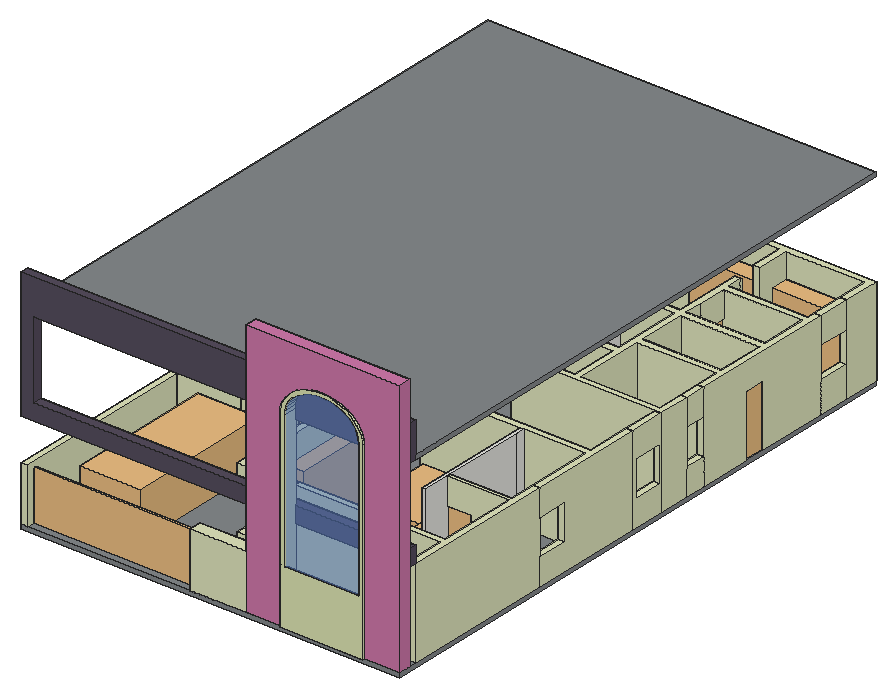
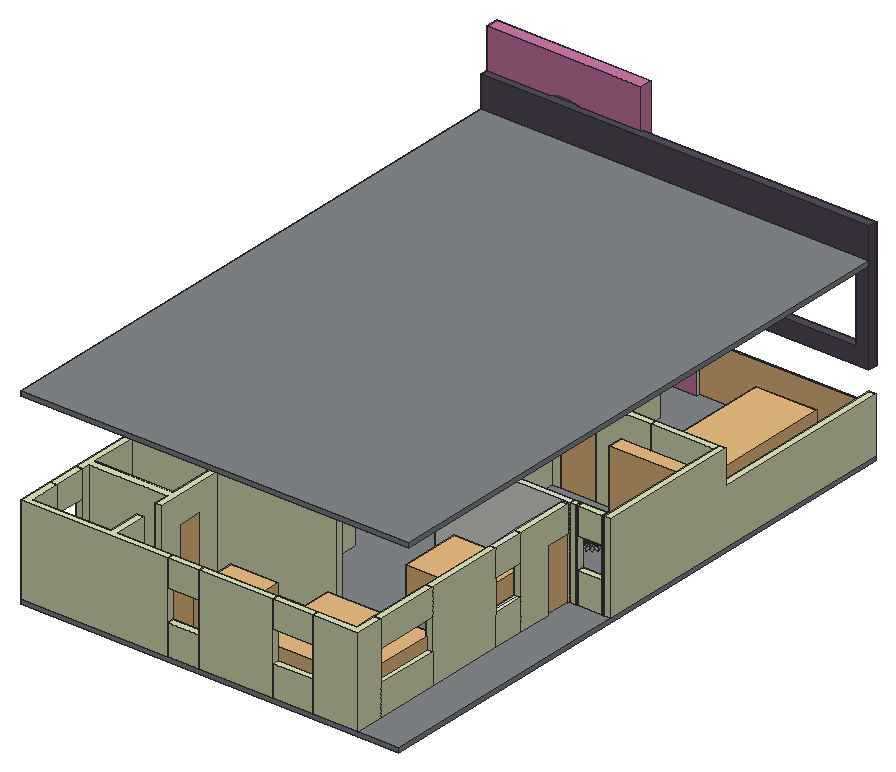
# SketchUp Ruby script. Lengths in inches.
U = 1.inch
M = Sketchup.active_model
def pt(a) = Geom::Point3d.new(a.map { |v| v * U })
def face(e, loops, mat)
  f = e.add_face(loops[0].map { |a| pt(a) })
  loops[1..].each { |l| e.add_face(l.map { |a| pt(a) }).erase! }
  f.material = f.back_material = mat if mat
  f
end
# faces: each face lists its corners as indices into pts; further lists are holes
def faces(e, pts, list, mat = nil) = list.each { |f| face(e, (f[0].is_a?(Array) ? f : [f]).map { |l| l.map { |i| pts[i] } }, mat) }
# xy, xz, yz: faces in a plane at the given z, y or x. An outline is a flat list of corners, or four numbers for a rectangle; further outlines are holes
def ring(l) = l.size == 4 ? [[l[0], l[1]], [l[2], l[1]], [l[2], l[3]], [l[0], l[3]]] : l.each_slice(2).to_a
def flat(e, list, mat, &to3) = list.each { |f| face(e, (f[0].is_a?(Array) ? f : [f]).map { |l| ring(l).map { |u, v| to3.(u, v) } }, mat) }
def xy(e, z, list, mat = nil) = flat(e, list, mat) { |x, y| [x, y, z] }
def xz(e, y, list, mat = nil) = flat(e, list, mat) { |x, z| [x, y, z] }
def yz(e, x, list, mat = nil) = flat(e, list, mat) { |y, z| [x, y, z] }
def lines(e, pts, list) = list.each { |a, b| e.add_line(pt(pts[a]), pt(pts[b])) }
# prism: a flat outline (further loops are holes) pulled along v
def prism(e, loops, v, mat = nil)
  f = face(e, loops, mat); d = Geom::Vector3d.new(v.map { |x| x * U })
  f.pushpull(f.normal.samedirection?(d) ? d.length : -d.length)
end
def box(e, o, s, mat = nil) = prism(e, [[o, [o[0] + s[0], o[1], o[2]], [o[0] + s[0], o[1] + s[1], o[2]], [o[0], o[1] + s[1], o[2]]]], [0, 0, s[2]], mat)
def at(x, y, z, deg = 0) = Geom::Transformation.translation(pt([x, y, z])) * Geom::Transformation.rotation(ORIGIN, Z_AXIS, deg.degrees)
def axes(o, x, y, z) = Geom::Transformation.new([*x, 0, *y, 0, *z, 0, *pt(o).to_a, 1])
def part(name) = M.definitions.add(name)
# library, detail: a bought-in or finely detailed component or shape, given as its bounding box
def library(name, o, s) = part(name).tap { |d| box(d.entities, o, s) }
def detail(e, o, s) = box(e.add_group.entities, o, s)
def put(e, d, t, mat = nil) = e.add_instance(d, t).tap { |i| i.material = mat if mat }
def group(e, t, mat = nil) = e.add_group.tap { |g| g.transformation = t; g.material = mat if mat }.entities
root = M.entities
M.materials.add("0206 AP 9414 PINK FLOWER").color = [207, 120, 170]
M.materials.add("0272 AP 9625 Blue Grape-N").color = [85, 77, 93]
M.materials.add("0748 AP 7713 LIME SQUASH").color = [220, 228, 179]
M.materials.add("0763 AP 7730 GREEN TOMATO").color = [223, 228, 188]
M.materials.add("0825 AP 9841 Aniseed Green-N").color = [202, 186, 112]
M.materials.add("[Blacktop Old 01]").color = [132, 136, 139]
M.materials.add("[Translucent Glass Blue]").color = [100, 149, 237]
M.materials["[Translucent Glass Blue]"].alpha = 0.5
c1 = library("michel-club1",[-34.67,-0.85,-0.13],[126.28,91.17,33.41])
c2 = library("Catia",[-24.7,0,-4.44],[60.13,63.39,38.33])
c3 = library("Mesa+de+Jantar+Clean-Ouro",[12.6875,-84.97,0.5625],[145.94,104.19,56.09])
c4 = library("toilet",[85.22,-15.77,0],[26.79,17.15,27.58])
c5 = library("bed",[0,0,0],[81.24,78.82,29.53])
c6 = library("Untitled",[0,0,0],[36,4.39,84])
c7 = part("Group\#146")
xy(c7.entities,0,[[0,0,18.2,28.93]])
xy(c7.entities,1.42,[[0.71,1.42,18.2,27.51]])
xy(c7.entities,13.47,[[0.71,1.42,18.2,27.51]])
xy(c7.entities,14.18,[[0.71,1.42,18.2,27.51]])
xy(c7.entities,25.88,[[0.71,1.42,18.2,27.51]])
xy(c7.entities,26.59,[[0.71,1.42,18.2,27.51]])
xy(c7.entities,38.65,[[0.71,1.42,18.2,27.51]])
xy(c7.entities,40.0625,[[0,0,18.2,28.93]])
xz(c7.entities,0,[[0,0,18.2,40.0625]])
xz(c7.entities,1.42,[[0.71,1.42,18.2,13.47],[0.71,14.18,18.2,25.88],[0.71,26.59,18.2,38.65]])
xz(c7.entities,27.51,[[0.71,1.42,18.2,13.47],[0.71,14.18,18.2,25.88],[0.71,26.59,18.2,38.65]])
xz(c7.entities,28.93,[[0,0,18.2,40.0625]])
yz(c7.entities,0,[[0,0,28.93,40.0625]])
yz(c7.entities,0.71,[[1.42,1.42,27.51,13.47],[1.42,14.18,27.51,25.88],[1.42,26.59,27.51,38.65]])
yz(c7.entities,18.2,[[[0,0,28.93,40.0625],[1.42,1.42,27.51,25.88],[1.42,26.59,27.51,38.65]],[1.42,13.47,27.51,14.18]])
c8 = library("tv unit model",[-7.7,0,0],[29.4,107.72,88.39])
c9 = part("*U2")
p = [[0,-10.98,0],[0.69,-9.51,0],[1.27,-7.99,0],[1.75,-6.43,0],[2.13,-4.85,0],[2.4,-3.25,0],
  [2.5625,-1.625,0],[2.62,0,0],[2.5625,1.625,0],[2.4,3.25,0],[2.13,4.85,0],[1.75,6.43,0],
  [1.27,7.99,0],[0.69,9.51,0],[0,10.98,0],[-0.69,9.51,0],[-1.27,7.99,0],[-1.75,6.43,0],
  [-2.13,4.85,0],[-2.4,3.25,0],[-2.5625,1.625,0],[-2.62,0,0],[-2.5625,-1.625,0],[-2.4,-3.25,0],
  [-2.13,-4.85,0],[-1.75,-6.43,0],[-1.27,-7.99,0],[-0.69,-9.51,0]]
lines(c9.entities,p,[[0,1],[1,2],[2,3],[3,4],[4,5],[5,6],[6,7],[7,8],[8,9],[9,10],[10,11],[11,12],
  [12,13],[13,14],[14,15],[15,16],[16,17],[17,18],[18,19],[19,20],[20,21],[21,22],[22,23],[23,24],
  [24,25],[25,26],[26,27],[27,0]])
c10 = part("*U3")
put(c10.entities,c9,at(0,11.05,0))
put(c10.entities,c9,at(-3.57,10.45,0,18.947))
put(c10.entities,c9,at(-6.74,8.73,0,37.895))
put(c10.entities,c9,at(-9.19,6.07,0,56.842))
put(c10.entities,c9,at(-10.65,2.76,0,75.789))
put(c10.entities,c9,at(-10.94,-0.84,0,94.737))
put(c10.entities,c9,at(-10.06,-4.35,0,113.684))
put(c10.entities,c9,at(-8.08,-7.37,0,132.632))
put(c10.entities,c9,at(-5.23,-9.59,0,151.579))
put(c10.entities,c9,at(-1.81,-10.77,0,170.526))
put(c10.entities,c9,at(1.81,-10.77,0,-170.526))
put(c10.entities,c9,at(5.23,-9.59,0,-151.579))
put(c10.entities,c9,at(8.08,-7.37,0,-132.632))
put(c10.entities,c9,at(10.06,-4.35,0,-113.684))
put(c10.entities,c9,at(10.94,-0.84,0,-94.737))
put(c10.entities,c9,at(10.65,2.76,0,-75.789))
put(c10.entities,c9,at(9.19,6.07,0,-56.842))
put(c10.entities,c9,at(6.74,8.73,0,-37.895))
put(c10.entities,c9,at(3.57,10.45,0,-18.947))
c11 = library("*U5",[-21.75,-13.5,0],[21,24,0.01])
c12 = library("Dining Set - 36 x 72 in.",[-45.5,-27.5,0],[91,55,0.01])
c13 = library("Range-Oven - 30 in top",[-15,-13,0],[30,26,0.01])
c14 = part("*U31")
p = [[-15.25,-21.5,0],[-17.25,-27.5,0],[-7.25,-27.5,0],[-15.25,-27.5,0]]
lines(c14.entities,p,[[0,1],[2,3]])
c15 = library("Component",[0,4.7,0],[98.27,23.62,86.61])
c16 = part("Group541\#1")
yz(c16.entities,285.5,[[630.18,36,645.93,59.625]])
c17 = library("Evoque+Azul+Marinho+As+Novinha+Fica+Loca+2017",[-10.19,-69.08,0],[168.96,82.02,63.04])
c18 = library("Table lamp",[7.65,497.27,0],[26.62,26.5,38.96])
c19 = library("Untitled\#1",[131.66,19.68,0],[2.41,197.25,46.46])
xy(root,0,[[46.9,331.33,68,331.34],[68,331.33,82.86,331.34],[68,531.6875,77,573.46]])
xy(root,42,[[68,531.6875,72.5,573.46],[72.5,531.6875,77,573.46]])
xy(root,84,[[68,531.6875,72.5,573.46],[72.5,531.6875,77,573.46]])
xy(root,120,[[68,531.6875,77,573.46]])
xz(root,531.6875,[[68,0,77,42],[72.5,42,77,84],[68,84,77,120]])
xz(root,573.46,[[68,0,77,42],[72.5,42,77,84],[68,84,77,120]])
yz(root,68,[[531.6875,0,573.46,42],[531.6875,84,573.46,120]],"0763 AP 7730 GREEN TOMATO")
yz(root,77,[[531.6875,0,573.46,42],[531.6875,84,573.46,120]])
g1 = group(root,at(13,81.3,-6),"[Blacktop Old 01]")
box(g1,[0,-79.3,0],[511,804.3,6])
put(root,c1,axes([138.46,548.07,-4.2],[0.78029,0,0],[0,-0.89729,0],[0,0,1.3]))
put(root,c2,at(358.59,682.03,1.34,90))
put(root,c3,axes([62.81,774.2,-1.46],[0.9696,0,0],[0,1.2019,0],[0,0,1.05545]))
put(root,c4,axes([538.71,590.5,-0.125],[-1.14901,0,0],[0,-1.05825,0],[0,0,0.99543]))
put(root,c5,axes([424.66,297.89,0],[-1.3,0,0],[0,-1.30842,0],[0,0,1.73]))
put(root,c6,at(402.09,693.8,0,-90))
put(root,c6,axes([431.91,202.21,0],[0.87201,0,0],[0,-1,0],[0,0,1]))
put(root,c6,at(70.09,486.39,0,-90))
put(root,c6,axes([517.09,585.65,0],[0,0.81291,0],[1,0,0],[0,0,1]))
put(root,c6,at(321.09,591.37,0,-90))
put(root,c6,axes([181,263.3,0],[1.33333,0,0],[0,-0.57478,0],[0,0,1]))
g2 = group(root,at(0,103.3,246.1875),"0763 AP 7730 GREEN TOMATO")
xy(g2,0,[[0,-74.28,524,703]],"[Blacktop Old 01]")
xy(g2,6,[[0,-74.28,524,703]],"[Blacktop Old 01]")
xz(g2,-101.3,[[369.99,-246.1875,470,-246.1875,470,13.0625,468.3,22.9,463.3,32.07,455.35,39.9375,445,45.98,432.9375,49.77,420,51.07,407.05,49.77,394.99,45.98,384.64,39.9375,376.69,32.07,371.7,22.9,369.99,13.0625]],"[Translucent Glass Blue]")
xz(g2,-74.28,[[18.41,0,524,6]])
xz(g2,703,[[0,0,524,6]],"[Blacktop Old 01]")
yz(g2,0,[[-74.28,0,703,6]],"[Blacktop Old 01]")
yz(g2,524,[[-74.28,0,703,6]],"[Blacktop Old 01]")
# 2 loose lines left out
g3 = group(g2,at(460.17,-84.3,-59.09))
xy(g3,-187.1,[[-96.18,-19,-96.18,-17,-219.17,-17,-219.17,0,-90.18,0,-90.18,-19],[-90.18,-19,-90.18,-17,9.83,-17,9.83,0,63.83,0,63.83,-17,15.83,-17,15.83,-19]])
xy(g3,-112.29,[[-90.18,-19,9.83,-17],[-219.17,-17,-144.18,0]])
xy(g3,160.3125,[[-144.18,-17,63.83,0]],"0206 AP 9414 PINK FLOWER")
xz(g3,-19,[[-96.18,-187.1,15.83,-187.1,15.83,72.15,15.35,77.71,13.92,83.17,11.56,88.4375,8.32,93.43,4.25,98.06,-0.58,102.25,-6.08,105.92,-12.17,109.01,-18.74,111.47,-25.68,113.26,-32.87,114.35,-40.18,114.71,-47.49,114.35,-54.67,113.26,-61.61,111.47,-68.18,109.01,-74.27,105.92,-79.78,102.25,-84.61,98.06,-88.68,93.43,-91.92,88.4375,-94.27,83.17,-95.7,77.71,-96.18,72.15,-96.18,-112.29,-90.18,-112.29,-90.18,72.15,-89.75,77.11,-88.48,81.99,-86.375,86.69,-83.48,91.15,-79.85,95.28,-75.53,99.02,-70.62,102.3,-65.18,105.0625,-59.3125,107.26,-53.12,108.86,-46.7,109.83,-40.18,110.15,-33.65,109.83,-27.23,108.86,-21.04,107.26,-15.17,105.0625,-9.74,102.3,-4.82,99.02,-0.51,95.28,3.13,91.15,6.02,86.69,8.125,81.99,9.4,77.11,9.83,72.15,9.83,-112.29,-96.18,-112.29]],"0748 AP 7713 LIME SQUASH")
xz(g3,-17,[[-219.17,-187.1,-144.18,-112.29],[-90.18,-187.1,9.83,-112.29]])
xz(g3,-17,[[-144.18,-187.1,-96.18,-187.1,-96.18,72.15,-95.7,77.71,-94.27,83.17,-91.92,88.4375,-88.68,93.43,-84.61,98.06,-79.78,102.25,-74.27,105.92,-68.18,109.01,-61.61,111.47,-54.67,113.26,-47.49,114.35,-40.18,114.71,-32.87,114.35,-25.68,113.26,-18.74,111.47,-12.17,109.01,-6.08,105.92,-0.58,102.25,4.25,98.06,8.32,93.43,11.56,88.4375,13.92,83.17,15.35,77.71,15.83,72.15,15.83,-187.1,63.83,-187.1,63.83,160.3125,-144.18,160.3125]],"0206 AP 9414 PINK FLOWER")
xz(g3,0,[[-219.17,-187.1,-219.17,-112.29,-144.18,-112.29,-144.18,160.3125,63.83,160.3125,63.83,-187.1,9.83,-187.1,9.83,72.15,9.4,77.11,8.125,81.99,6.02,86.69,3.13,91.15,-0.51,95.28,-4.82,99.02,-9.74,102.3,-15.17,105.0625,-21.04,107.26,-27.23,108.86,-33.65,109.83,-40.18,110.15,-46.7,109.83,-53.12,108.86,-59.3125,107.26,-65.18,105.0625,-70.62,102.3,-75.53,99.02,-79.85,95.28,-83.48,91.15,-86.375,86.69,-88.48,81.99,-89.75,77.11,-90.18,72.15,-90.18,-187.1]],"0206 AP 9414 PINK FLOWER")
yz(g3,-219.17,[[-17,-187.1,0,-112.29]])
yz(g3,-144.18,[[-17,-112.29,0,160.3125]],"0206 AP 9414 PINK FLOWER")
yz(g3,-96.18,[[-19,-187.1,-17,72.15]])
yz(g3,-90.18,[[-17,-187.1,0,-187.1,0,72.15,-19,72.15,-19,-112.29,-17,-112.29]])
yz(g3,9.83,[[-17,-187.1,-17,-112.29,-19,-112.29,-19,72.15,0,72.15,0,-187.1]])
yz(g3,15.83,[[-19,-187.1,-17,72.15]])
yz(g3,63.83,[[-17,-187.1,0,160.3125]],"0206 AP 9414 PINK FLOWER")
p = [[-95.7,-17,77.71],[-96.18,-17,72.15],[-96.18,-19,72.15],[-95.7,-19,77.71],[-89.75,0,77.11],[-89.75,-19,77.11],
  [-90.18,-19,72.15],[-90.18,0,72.15],[9.83,0,72.15],[9.83,-19,72.15],[9.4,-19,77.11],[9.4,0,77.11],
  [15.83,-17,72.15],[15.35,-17,77.71],[15.35,-19,77.71],[15.83,-19,72.15],[-88.48,0,81.99],[-88.48,-19,81.99],
  [8.125,-19,81.99],[8.125,0,81.99],[-94.27,-17,83.17],[-94.27,-19,83.17],[13.92,-17,83.17],[13.92,-19,83.17],
  [-86.375,0,86.69],[-86.375,-19,86.69],[6.02,-19,86.69],[6.02,0,86.69],[-91.92,-17,88.4375],[-91.92,-19,88.4375],
  [11.56,-17,88.4375],[11.56,-19,88.4375],[-83.48,0,91.15],[-83.48,-19,91.15],[3.13,-19,91.15],[3.13,0,91.15],
  [-88.68,-17,93.43],[-88.68,-19,93.43],[8.32,-17,93.43],[8.32,-19,93.43],[-79.85,0,95.28],[-79.85,-19,95.28],
  [-0.51,-19,95.28],[-0.51,0,95.28],[-84.61,-17,98.06],[-84.61,-19,98.06],[4.25,-17,98.06],[4.25,-19,98.06],
  [-75.53,0,99.02],[-75.53,-19,99.02],[-4.82,-19,99.02],[-4.82,0,99.02],[-79.78,-17,102.25],[-79.78,-19,102.25],
  [-0.58,-17,102.25],[-0.58,-19,102.25],[-70.62,0,102.3],[-70.62,-19,102.3],[-9.74,-19,102.3],[-9.74,0,102.3],
  [-74.27,-17,105.92],[-74.27,-19,105.92],[-6.08,-17,105.92],[-6.08,-19,105.92],[-65.18,0,105.0625],[-65.18,-19,105.0625],
  [-15.17,-19,105.0625],[-15.17,0,105.0625],[-59.3125,0,107.26],[-59.3125,-19,107.26],[-21.04,-19,107.26],[-21.04,0,107.26],
  [-68.18,-17,109.01],[-68.18,-19,109.01],[-12.17,-17,109.01],[-12.17,-19,109.01],[-53.12,0,108.86],[-53.12,-19,108.86],
  [-27.23,-19,108.86],[-27.23,0,108.86],[-46.7,0,109.83],[-46.7,-19,109.83],[-33.65,-19,109.83],[-33.65,0,109.83],
  [-61.61,-17,111.47],[-61.61,-19,111.47],[-18.74,-17,111.47],[-18.74,-19,111.47],[-40.18,0,110.15],[-40.18,-19,110.15],
  [-54.67,-17,113.26],[-54.67,-19,113.26],[-25.68,-17,113.26],[-25.68,-19,113.26],[-47.49,-17,114.35],[-47.49,-19,114.35],
  [-32.87,-17,114.35],[-32.87,-19,114.35],[-40.18,-17,114.71],[-40.18,-19,114.71]]
faces(g3,p,[[0,1,2,3],[4,5,6,7],[8,9,10,11],[12,13,14,15],[16,17,5,4],[11,10,18,19],[20,0,3,21],[13,22,23,14],
  [24,25,17,16],[19,18,26,27],[28,20,21,29],[22,30,31,23],[32,33,25,24],[27,26,34,35],[36,28,29,37],[30,38,39,31],
  [40,41,33,32],[35,34,42,43],[44,36,37,45],[38,46,47,39],[48,49,41,40],[43,42,50,51],[52,44,45,53],[46,54,55,47],
  [56,57,49,48],[51,50,58,59],[60,52,53,61],[54,62,63,55],[64,65,57,56],[59,58,66,67],[68,69,65,64],[67,66,70,71],
  [72,60,61,73],[62,74,75,63],[76,77,69,68],[71,70,78,79],[80,81,77,76],[79,78,82,83],[84,72,73,85],[74,86,87,75],
  [88,89,81,80],[83,82,89,88],[90,84,85,91],[86,92,93,87],[94,90,91,95],[92,96,97,93],[98,94,95,99],[96,98,99,97]])
g4 = group(g2,at(0,-74.28,0))
prism(g4,[[[524,0,-126.1875],[0,0,-126.1875],[0,0,47.75],[524,0,47.75],[524,0,0],[18.41,0,0],[18.41,0,-103.72],[524,0,-103.72]]],[0,-12,0],"0272 AP 9625 Blue Grape-N")
put(root,c7,axes([515,584.23,40.0625],[-1,0,0],[0,-1,0],[0,0,-1]))
put(root,c8,axes([265.34,277.74,0],[-1,0,0],[0,-1.15462,0],[0,0,1]))
put(root,c8,axes([39.42,277.11,0],[0,-0.89,0],[1,0,0],[0,0,1]))
put(root,c10,at(130.65,333.16,0))
put(root,c11,at(221.36,413.43,0))
put(root,c12,at(148.3,730.4,0))
put(root,c13,at(371.81,784.32,0))
put(root,c13,at(489.86,784,0))
put(root,c14,axes([395.6,587.5,0],[0,-1,0],[-1,0,0],[0,0,1]))
put(root,c15,axes([395.71,768.58,0],[-1,0,0],[0,1,0],[0,0,1]))
put(root,c15,axes([515,768.58,0],[-1.07869,0,0],[0,1,0],[0,0,1]))
g5 = group(root,at(183.44,797.3,0),"0763 AP 7730 GREEN TOMATO")
box(g5,[0,0,0],[99.53,9,120])
g6 = group(root,at(68,486.39,0),"0763 AP 7730 GREEN TOMATO")
prism(g6,[[[0,45.3,0],[0,0,0],[0,0,84],[0,-34.09,84],[0,-34.09,120],[0,45.3,120]]],[9,0,0])
g7 = group(root,at(68,768.52,0),"0763 AP 7730 GREEN TOMATO")
prism(g7,[[[0,37.78,0],[61.44,37.78,0],[61.44,28.78,0],[9,28.78,0],[9,0,0],[0,0,0]]],[0,0,120])
g8 = group(root,at(324.97,752.73,0),"0763 AP 7730 GREEN TOMATO")
prism(g8,[[[199.03,53.57,0],[199.03,3.1,0],[190.03,3.1,0],[190.03,44.57,0],[84.03,44.57,0],[84.03,0,0],[75.03,0,0],[75.03,44.57,0],[0,44.57,0],[0,53.57,0]]],[0,0,120])
g9 = group(root,at(229,170.7,0),"0763 AP 7730 GREEN TOMATO")
xy(g9,0,[[12,0,12,83.61,0,83.61,0,92.61,12,92.61,12,164.61,27,164.61,27,155.61,21,155.61,21,0]])
xy(g9,84,[[-48,83.61,0,92.61]])
xy(g9,120,[[12,0,21,0,21,155.61,27,155.61,27,164.61,12,164.61,12,92.61,-48,92.61,-48,83.61,12,83.61]])
xz(g9,0,[[12,0,17,120],[17,0,21,120]])
xz(g9,83.61,[[0,0,12,0,12,120,-48,120,-48,84,0,84]])
xz(g9,92.61,[[0,0,0,84,-48,84,-48,120,12,120,12,0]])
xz(g9,155.61,[[21,0,27,120]])
xz(g9,164.61,[[12,0,27,120]])
yz(g9,-48,[[83.61,84,92.61,120]])
yz(g9,0,[[83.61,0,92.61,84]])
yz(g9,12,[[0,0,83.61,120],[92.61,0,164.61,120]])
yz(g9,21,[[0,0,155.61,120]])
yz(g9,27,[[155.61,0,164.61,120]])
g10 = group(root,at(427,161.21,0))
prism(g10,[[[0,165.1,0],[5,165.1,0],[5,152.78,0],[5,0,0],[0,0,0]]],[0,0,120])
g11 = group(root,at(107.4,254.3,0),"0763 AP 7730 GREEN TOMATO")
prism(g11,[[[73.6,0,0],[0,0,0],[0,4.44,0],[0,9,0],[73.6,9,0]]],[0,0,120])
g12 = group(root,at(22,440.3,0),"0825 AP 9841 Aniseed Green-N")
box(g12,[0,0,0],[3,9,120])
g13 = group(root,at(13,254.3,0),"0763 AP 7730 GREEN TOMATO")
xy(g13,0,[[0,-252.3,9,195]])
xy(g13,74.8125,[[0,-252.3,9,0]])
xy(g13,120,[[0,0,9,195]])
xz(g13,-252.3,[[0,0,9,74.8125]])
xz(g13,0,[[0,74.8125,9,120]])
xz(g13,195,[[0,0,9,120]])
yz(g13,0,[[-252.3,0,-252.3,74.8125,0,74.8125,0,120,195,120,195,0]])
yz(g13,9,[[-252.3,0,9,0,9,120,0,120,0,74.8125,-252.3,74.8125],[9,0,186,120],[186,0,195,120]])
g14 = group(root,at(68,449.3,0),"0763 AP 7730 GREEN TOMATO")
prism(g14,[[[0,3,0],[9,3,0],[9,0,0],[4.5,0,0],[0,0,0]]],[0,0,120])
g15 = group(root,at(68,440.3,0))
prism(g15,[[[182,0,0],[0,0,0],[0,9,0],[4.5,9,0],[9,9,0],[182,9,0]]],[0,0,120])
g16 = group(root,at(129.44,797.3,0),"0763 AP 7730 GREEN TOMATO")
box(g16,[0,0,0],[54,9,42])
box(g16,[0,0,84],[54,9,36])
# 2 loose lines left out
g17 = group(root,at(60.38,440.3,0),"0763 AP 7730 GREEN TOMATO")
box(g17,[0,0,0],[7.62,9,120])
g18 = group(root,at(282.97,797.3,0),"0763 AP 7730 GREEN TOMATO")
box(g18,[0,0,0],[42,9,42])
box(g18,[0,0,84],[42,9,36])
# 2 loose lines left out
g19 = group(root,at(238.5,443.3,0),"0763 AP 7730 GREEN TOMATO")
xy(g19,0,[[82.5,0,82.5,21.03,91.5,21.03,91.5,9,161.5,9,161.5,74,91.5,74,91.5,52.96,82.5,52.96,82.5,83,161.5,83,161.5,177,0,177,0,186,161.5,186,161.5,214.5,170.5,214.5,170.5,186.08,276.5,186.08,276.5,249,161.5,249,161.5,279.43,170.5,279.43,170.5,258,276.5,258,276.5,269.19,285.5,269.19,285.5,171.61,276.5,171.61,276.5,177,170.5,177,170.5,112,276.5,112,276.5,142.35,285.5,142.35,285.5,72.02,276.5,72.02,276.5,103,170.5,103,170.5,9,276.5,9,276.5,43.72,285.5,43.72,285.5,0]])
xy(g19,84,[[276.5,142.35,285.5,171.61],[161.5,214.5,170.5,249]])
xy(g19,120,[[[82.5,0,285.5,0,285.5,43.72,276.5,43.72,276.5,9,170.5,9,170.5,103,276.5,103,276.5,72.02,285.5,72.02,285.5,269.19,276.5,269.19,276.5,258,170.5,258,170.5,279.43,161.5,279.43,161.5,186,0,186,0,177,161.5,177,161.5,83,82.5,83,82.5,52.96,91.5,52.96,91.5,74,161.5,74,161.5,9,91.5,9,91.5,21.03,82.5,21.03],[170.5,112,276.5,177],[170.5,186.08,276.5,249]]])
xz(g19,0,[[82.5,0,281.65,120],[281.65,0,285.5,120]])
xz(g19,9,[[91.5,0,161.5,120],[170.5,0,276.5,120]])
xz(g19,21.03,[[82.5,0,91.5,120]])
xz(g19,43.72,[[276.5,0,285.5,120]])
xz(g19,52.96,[[82.5,0,91.5,120]])
xz(g19,72.02,[[276.5,0,285.5,120]])
xz(g19,74,[[91.5,0,161.5,120]])
xz(g19,83,[[82.5,0,161.5,120]])
xz(g19,103,[[170.5,0,276.5,120]])
xz(g19,112,[[170.5,0,276.5,120]])
xz(g19,142.35,[[276.5,0,285.5,84]])
xz(g19,171.61,[[276.5,0,285.5,84]])
xz(g19,177,[[0,0,161.5,120],[170.5,0,276.5,120]])
xz(g19,186,[[0,0,161.5,120]])
xz(g19,186.08,[[170.5,0,276.5,120]])
xz(g19,214.5,[[161.5,0,170.5,84]])
xz(g19,249,[[161.5,0,276.5,0,276.5,120,170.5,120,170.5,84,161.5,84]])
xz(g19,258,[[170.5,0,276.5,120]])
xz(g19,269.19,[[276.5,0,285.5,120]])
xz(g19,279.43,[[161.5,0,170.5,120]])
yz(g19,0,[[177,0,186,120]])
yz(g19,82.5,[[0,0,21.03,120],[52.96,0,83,120]])
yz(g19,91.5,[[9,0,21.03,120],[52.96,0,74,120]])
yz(g19,161.5,[[9,0,74,120],[83,0,177,120],[186,0,186,120,279.43,120,279.43,0,249,0,249,84,214.5,84,214.5,0]])
yz(g19,170.5,[[9,0,103,120],[112,0,177,120],[186.08,0,210.08,120],[210.08,0,214.5,0,214.5,84,249,84,249,120,210.08,120],[258,0,276.99,120],
  [276.99,0,279.43,120]])
yz(g19,276.5,[[9,0,43.72,120],[72.02,0,103,120],[112,0,112,120,177,120,177,0,171.61,0,171.61,84,142.35,84,142.35,0],[186.08,0,249,120],[258,0,269.19,120]])
yz(g19,285.5,[[0,0,43.72,120],[72.02,0,142.35,0,142.35,84,171.61,84,171.61,0,269.19,0,269.19,120,72.02,120]])
g20 = group(root,at(321,591.37,0))
prism(g20,[[[5,0,0],[5,28.93,0],[5,28.93,120],[5,-30.46,120],[5,-30.46,84],[5,0,84]]],[-5,0,0])
g21 = group(root,at(321,526.3,0))
box(g21,[0,0,0],[5,34.61,120])
put(root,c7,at(326,591.37,0))
g22 = group(root,at(515,487.02,0),"0763 AP 7730 GREEN TOMATO")
prism(g22,[[[9,0,84],[0,0,84],[0,28.29,84],[4.82,28.29,84],[9,28.29,84]]],[0,0,36])
xy(g22,36,[[0,0,9,28.29]])
xz(g22,0,[[0,0,9,36]])
xz(g22,28.29,[[0,0,9,36]])
yz(g22,0,[[0,0,28.29,36]])
yz(g22,9,[[0,0,28.29,36]])
# 2 loose lines left out
put(g22,c16,at(-726.875,-630.18,0))
g23 = group(root,at(292,280.53,0),"0763 AP 7730 GREEN TOMATO")
xy(g23,0,[[223,-42,223,45.77,0,45.77,0,54.77,223,54.77,223,114.77,232,114.77,232,-42]])
xy(g23,36,[[223,-42,232,0]])
xy(g23,84,[[223,-42,232,0]])
xy(g23,120,[[223,-42,232,-42,232,114.77,223,114.77,223,54.77,0,54.77,0,45.77,223,45.77]])
xz(g23,-42,[[223,0,232,36],[223,84,232,120]])
xz(g23,0,[[223,36,232,84]])
xz(g23,45.77,[[0,0,135,120],[135,0,140,120],[140,0,223,120]])
xz(g23,54.77,[[0,0,223,120]])
xz(g23,114.77,[[223,0,228.15,120],[228.15,0,232,120]])
yz(g23,0,[[45.77,0,54.77,120]])
yz(g23,223,[[-42,0,-42,36,0,36,0,84,-42,84,-42,120,45.77,120,45.77,0],[54.77,0,114.77,120]])
yz(g23,232,[[-42,0,114.77,0,114.77,120,-42,120,-42,84,0,84,0,36,-42,36]])
g24 = group(root,at(520.15,395.3,0),"0763 AP 7730 GREEN TOMATO")
prism(g24,[[[3.85,0,0],[3.85,48,0],[3.85,48,120],[3.85,0,120]],[[3.85,5.0625,84],[3.85,46,84],[3.85,46,36],[3.85,5.0625,36]]],[-9,0,0])
g25 = group(root,at(246,86.3,0),"0763 AP 7730 GREEN TOMATO")
xy(g25,0,[[-5,-5,-5,84.39,4,84.39,4,4,72.49,4,72.49,-5]])
xy(g25,36,[[-5,-5,72.49,-5,72.49,4,4,4,4,59.55,-5,59.55]])
xy(g25,84,[[-5,-5,-5,59.55,4,59.55,4,4,72.49,4,72.49,-5]])
xy(g25,120,[[-5,-5,72.49,-5,72.49,4,4,4,4,84.39,-5,84.39]])
xz(g25,-5,[[-5,0,72.49,36],[-5,84,72.49,120]])
xz(g25,4,[[4,0,72.49,36],[4,84,72.49,120]])
xz(g25,59.55,[[-5,36,4,84]])
xz(g25,84.39,[[-5,0,4,120]])
yz(g25,-5,[[-5,0,84.39,36],[59.55,36,84.39,84],[-5,84,84.39,120]])
yz(g25,4,[[4,0,84.39,0,84.39,120,4,120,4,84,59.55,84,59.55,36,4,36]])
yz(g25,72.49,[[-5,0,4,36],[-5,84,4,120]])
# 1 loose lines left out
g26 = group(root,at(22,254.3,0),"0763 AP 7730 GREEN TOMATO")
prism(g26,[[[85.4,9,0],[85.4,4.44,0],[85.4,0,0],[0,0,0],[0,9,0]]],[0,0,120])
g27 = group(root,at(57.38,440.3,0),"0763 AP 7730 GREEN TOMATO")
box(g27,[0,0,0],[3,9,120])
g28 = group(root,at(25,445.11,0),"0763 AP 7730 GREEN TOMATO")
box(g28,[0,-4.81,0],[32.38,9,42])
box(g28,[0,-4.81,84.0625],[32.38,9,35.9375])
# 2 loose lines left out
g29 = group(root,at(68,680.93,0),"0763 AP 7730 GREEN TOMATO")
prism(g29,[[[0,0,0],[0,87.59,0],[9,87.59,0],[9,84.59,0],[9,3,0],[9,0,0]]],[0,0,42])
prism(g29,[[[0,0,84],[0,87.59,84],[9,87.59,84],[9,84.59,84],[9,3,84],[9,0,84]]],[0,0,36])
# 2 loose lines left out
g30 = group(root,at(68,573.46,0),"0763 AP 7730 GREEN TOMATO")
box(g30,[0,0,0],[9,107.47,120])
g31 = group(root,at(519,712.5,0),"0763 AP 7730 GREEN TOMATO")
box(g31,[-4,0,0],[9,43.33,42])
box(g31,[-4,0,84],[9,43.33,36])
# 2 loose lines left out
g32 = group(root,at(318.49,47.13,0),"0763 AP 7730 GREEN TOMATO")
xy(g32,0,[[196.51,-18.11,196.51,34.17,0,34.17,0,43.17,108.51,43.17,108.51,67.17,113.51,67.17,113.51,43.17,196.51,43.17,196.51,150.17,144.81,150.17,144.81,155.17,196.51,155.17,196.51,191.39,205.51,191.39,205.51,-18.11]])
xy(g32,84,[[113.51,150.17,144.81,155.17]])
xy(g32,120,[[196.51,-18.11,205.51,-18.11,205.51,191.39,196.51,191.39,196.51,155.17,113.51,155.17,113.51,150.17,196.51,150.17,196.51,43.17,113.51,43.17,113.51,67.17,108.51,67.17,108.51,43.17,0,43.17,0,34.17,196.51,34.17]])
xz(g32,-18.11,[[196.51,0,205.51,120]])
xz(g32,34.17,[[0,0,196.51,120]])
xz(g32,43.17,[[0,0,108.51,120],[113.51,0,196.51,120]])
xz(g32,67.17,[[108.51,0,113.51,120]])
xz(g32,150.17,[[144.81,0,196.51,0,196.51,120,113.51,120,113.51,84,144.81,84]])
xz(g32,155.17,[[144.81,0,144.81,84,113.51,84,113.51,120,196.51,120,196.51,0]])
xz(g32,191.39,[[196.51,0,205.51,120]])
yz(g32,0,[[34.17,0,43.17,120]])
yz(g32,108.51,[[43.17,0,67.17,120]])
yz(g32,113.51,[[43.17,0,67.17,120],[150.17,84,155.17,120]])
yz(g32,144.81,[[150.17,0,155.17,84]])
yz(g32,196.51,[[-18.11,0,34.17,120],[43.17,0,150.17,120],[155.17,0,191.39,120]])
yz(g32,205.51,[[-18.11,0,191.39,120]])
put(root,c17,axes([65.43,63.88,0],[0,1.17972,0],[-1,0,0],[0,0,1]))
put(root,c4,axes([269.83,606.61,0],[1.14901,0,0],[0,1.05825,0],[0,0,0.99543]))
put(root,c18,axes([392.73,-318.86,0],[1,0,0],[0,1,0],[0,0,1.41]))
put(root,c18,at(392.73,-210.67,0))
put(root,c19,axes([262.86,-119.44,0],[0,1,0],[-1.1103,0,0],[0,0,1.47]))
